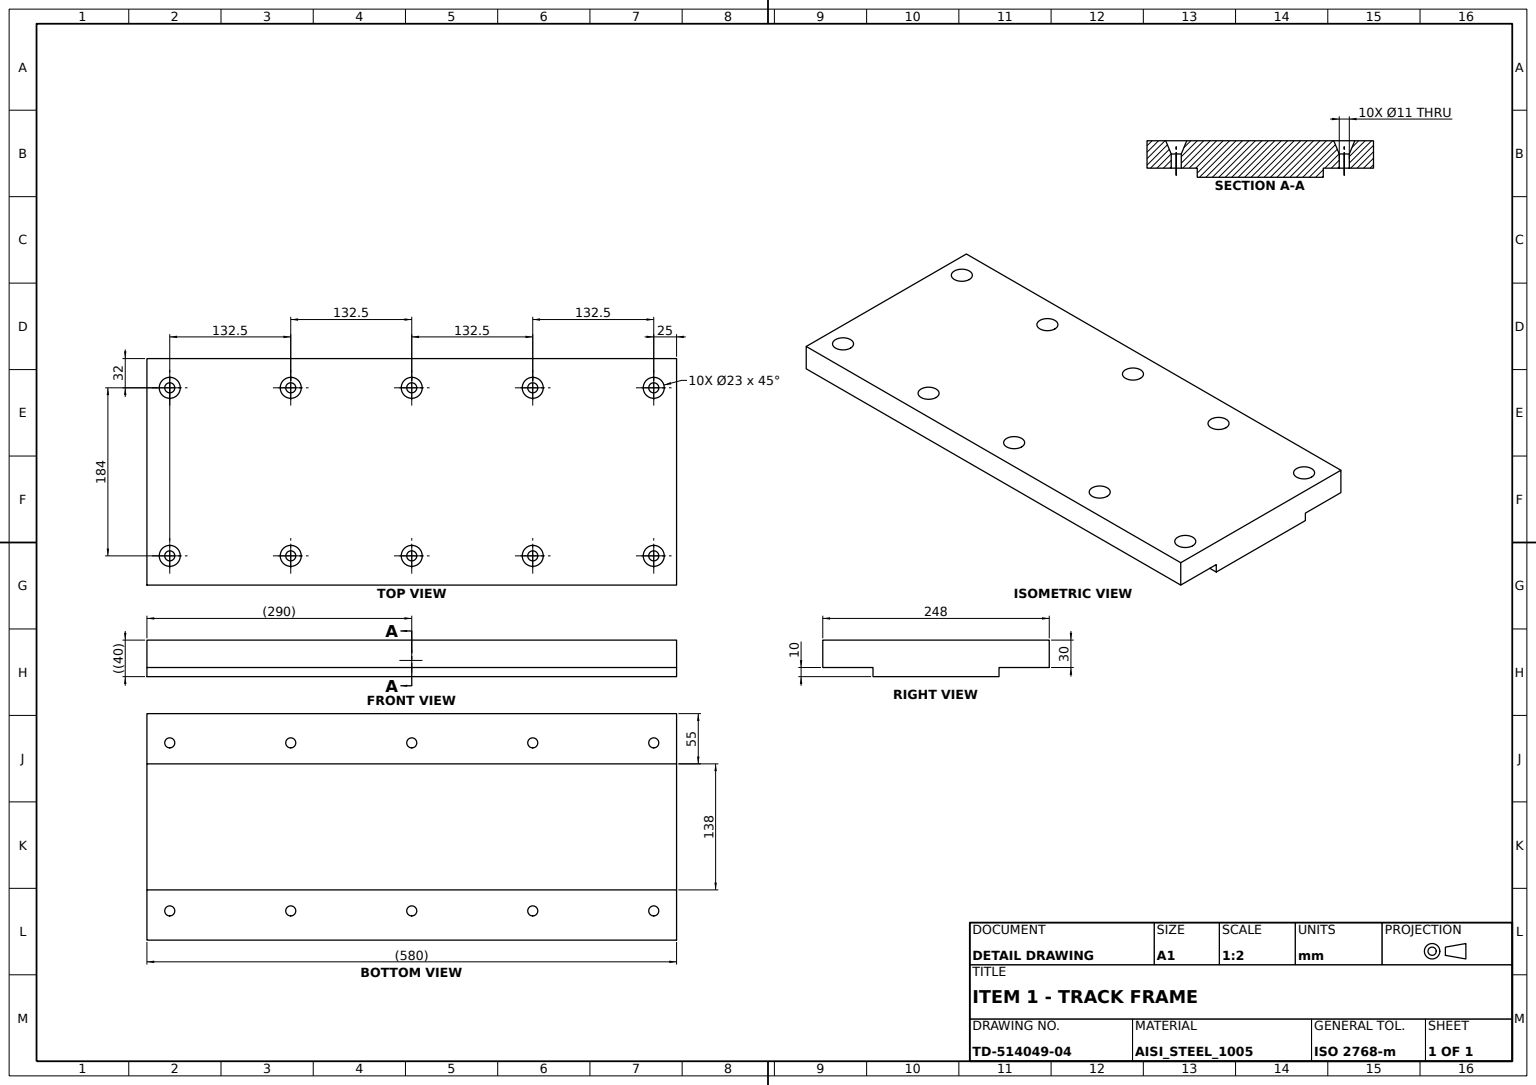
ISO-10303-21;
HEADER;
FILE_DESCRIPTION((''),'2;1');
FILE_NAME('','',(''),(''),'','','');
FILE_SCHEMA(('AUTOMOTIVE_DESIGN'));
ENDSEC;
DATA;
#1=APPLICATION_CONTEXT('');
#2=PRODUCT_CONTEXT('',#1,'mechanical');
#3=PRODUCT('','','',(#2));
#4=PRODUCT_DEFINITION_FORMATION('','',#3);
#5=PRODUCT_DEFINITION_CONTEXT('',#1,'design');
#6=PRODUCT_DEFINITION('','',#4,#5);
#7=PRODUCT_DEFINITION_SHAPE('','',#6);
#8=(LENGTH_UNIT()NAMED_UNIT(*)SI_UNIT(.MILLI.,.METRE.));
#9=(NAMED_UNIT(*)PLANE_ANGLE_UNIT()SI_UNIT($,.RADIAN.));
#10=(NAMED_UNIT(*)SI_UNIT($,.STERADIAN.)SOLID_ANGLE_UNIT());
#11=UNCERTAINTY_MEASURE_WITH_UNIT(LENGTH_MEASURE(0.005),#8,'distance_accuracy_value','');
#12=(GEOMETRIC_REPRESENTATION_CONTEXT(3)GLOBAL_UNCERTAINTY_ASSIGNED_CONTEXT((#11))GLOBAL_UNIT_ASSIGNED_CONTEXT((#8,#9,#10))REPRESENTATION_CONTEXT('',''));
#13=CARTESIAN_POINT('',(-97.5,0.,-132.5));
#14=VERTEX_POINT('',#13);
#15=CARTESIAN_POINT('',(-92.,0.,-132.5));
#16=DIRECTION('',(0.,1.,0.));
#17=DIRECTION('',(-1.,0.,0.));
#18=AXIS2_PLACEMENT_3D('',#15,#16,#17);
#19=CIRCLE('',#18,5.5);
#20=EDGE_CURVE('',#14,#14,#19,.T.);
#21=ORIENTED_EDGE('',*,*,#20,.F.);
#22=EDGE_LOOP('',(#21));
#23=FACE_BOUND('',#22,.T.);
#24=CARTESIAN_POINT('',(-92.,15.514719,-138.));
#25=VERTEX_POINT('',#24);
#26=CARTESIAN_POINT('',(-92.,15.514719,-132.5));
#27=DIRECTION('',(0.,-1.,0.));
#28=DIRECTION('',(0.,0.,-1.));
#29=AXIS2_PLACEMENT_3D('',#26,#27,#28);
#30=CIRCLE('',#29,5.5);
#31=EDGE_CURVE('',#25,#25,#30,.F.);
#32=ORIENTED_EDGE('',*,*,#31,.T.);
#33=EDGE_LOOP('',(#32));
#34=FACE_BOUND('',#33,.T.);
#35=CARTESIAN_POINT('',(-92.,-494999.973717,-132.5));
#36=AXIS2_PLACEMENT_3D('',#35,#27,#28);
#37=CYLINDRICAL_SURFACE('',#36,5.5);
#38=ADVANCED_FACE('',(#23,#34),#37,.F.);
#39=CARTESIAN_POINT('',(92.,15.514719,259.5));
#40=VERTEX_POINT('',#39);
#41=CARTESIAN_POINT('',(92.,15.514719,265.));
#42=AXIS2_PLACEMENT_3D('',#41,#27,#28);
#43=CIRCLE('',#42,5.5);
#44=EDGE_CURVE('',#40,#40,#43,.F.);
#45=ORIENTED_EDGE('',*,*,#44,.F.);
#46=EDGE_LOOP('',(#45));
#47=FACE_BOUND('',#46,.T.);
#48=CARTESIAN_POINT('',(92.,30.,253.5));
#49=VERTEX_POINT('',#48);
#50=CARTESIAN_POINT('',(92.,30.,265.));
#51=AXIS2_PLACEMENT_3D('',#50,#27,#28);
#52=CIRCLE('',#51,11.5);
#53=EDGE_CURVE('',#49,#49,#52,.T.);
#54=ORIENTED_EDGE('',*,*,#53,.F.);
#55=EDGE_LOOP('',(#54));
#56=FACE_BOUND('',#55,.T.);
#57=DIRECTION('',(0.,0.,1.));
#58=AXIS2_PLACEMENT_3D('',#50,#16,#57);
#59=CONICAL_SURFACE('',#58,11.5,0.392699082);
#60=ADVANCED_FACE('',(#47,#56),#59,.F.);
#61=CARTESIAN_POINT('',(92.,15.514719,-138.));
#62=VERTEX_POINT('',#61);
#63=CARTESIAN_POINT('',(92.,15.514719,-132.5));
#64=AXIS2_PLACEMENT_3D('',#63,#27,#28);
#65=CIRCLE('',#64,5.5);
#66=EDGE_CURVE('',#62,#62,#65,.F.);
#67=ORIENTED_EDGE('',*,*,#66,.F.);
#68=EDGE_LOOP('',(#67));
#69=FACE_BOUND('',#68,.T.);
#70=CARTESIAN_POINT('',(92.,30.,-144.));
#71=VERTEX_POINT('',#70);
#72=CARTESIAN_POINT('',(92.,30.,-132.5));
#73=AXIS2_PLACEMENT_3D('',#72,#27,#28);
#74=CIRCLE('',#73,11.5);
#75=EDGE_CURVE('',#71,#71,#74,.T.);
#76=ORIENTED_EDGE('',*,*,#75,.F.);
#77=EDGE_LOOP('',(#76));
#78=FACE_BOUND('',#77,.T.);
#79=AXIS2_PLACEMENT_3D('',#72,#16,#57);
#80=CONICAL_SURFACE('',#79,11.5,0.392699082);
#81=ADVANCED_FACE('',(#69,#78),#80,.F.);
#82=CARTESIAN_POINT('',(86.5,0.,132.5));
#83=VERTEX_POINT('',#82);
#84=CARTESIAN_POINT('',(92.,0.,132.5));
#85=AXIS2_PLACEMENT_3D('',#84,#16,#17);
#86=CIRCLE('',#85,5.5);
#87=EDGE_CURVE('',#83,#83,#86,.T.);
#88=ORIENTED_EDGE('',*,*,#87,.F.);
#89=EDGE_LOOP('',(#88));
#90=FACE_BOUND('',#89,.T.);
#91=CARTESIAN_POINT('',(92.,15.514719,127.));
#92=VERTEX_POINT('',#91);
#93=CARTESIAN_POINT('',(92.,15.514719,132.5));
#94=AXIS2_PLACEMENT_3D('',#93,#27,#28);
#95=CIRCLE('',#94,5.5);
#96=EDGE_CURVE('',#92,#92,#95,.F.);
#97=ORIENTED_EDGE('',*,*,#96,.T.);
#98=EDGE_LOOP('',(#97));
#99=FACE_BOUND('',#98,.T.);
#100=CARTESIAN_POINT('',(92.,-494999.973717,132.5));
#101=AXIS2_PLACEMENT_3D('',#100,#27,#28);
#102=CYLINDRICAL_SURFACE('',#101,5.5);
#103=ADVANCED_FACE('',(#90,#99),#102,.F.);
#104=CARTESIAN_POINT('',(124.,0.,290.));
#105=VERTEX_POINT('',#104);
#106=CARTESIAN_POINT('',(124.,30.,290.));
#107=VERTEX_POINT('',#106);
#108=VECTOR('',#16,1000.);
#109=LINE('',#104,#108);
#110=EDGE_CURVE('',#105,#107,#109,.T.);
#111=ORIENTED_EDGE('',*,*,#110,.F.);
#112=CARTESIAN_POINT('',(124.,0.,-290.));
#113=VERTEX_POINT('',#112);
#114=VECTOR('',#28,1000.);
#115=LINE('',#104,#114);
#116=EDGE_CURVE('',#105,#113,#115,.T.);
#117=ORIENTED_EDGE('',*,*,#116,.T.);
#118=CARTESIAN_POINT('',(124.,30.,-290.));
#119=VERTEX_POINT('',#118);
#120=LINE('',#112,#108);
#121=EDGE_CURVE('',#113,#119,#120,.T.);
#122=ORIENTED_EDGE('',*,*,#121,.T.);
#123=LINE('',#106,#114);
#124=EDGE_CURVE('',#107,#119,#123,.T.);
#125=ORIENTED_EDGE('',*,*,#124,.F.);
#126=EDGE_LOOP('',(#111,#117,#122,#125));
#127=FACE_BOUND('',#126,.T.);
#128=AXIS2_PLACEMENT_3D('',#104,#17,#57);
#129=PLANE('',#128);
#130=ADVANCED_FACE('',(#127),#129,.F.);
#131=CARTESIAN_POINT('',(-69.,0.,-290.));
#132=VERTEX_POINT('',#131);
#133=CARTESIAN_POINT('',(-69.,-10.,-290.));
#134=VERTEX_POINT('',#133);
#135=VECTOR('',#27,1000.);
#136=LINE('',#131,#135);
#137=EDGE_CURVE('',#132,#134,#136,.T.);
#138=ORIENTED_EDGE('',*,*,#137,.T.);
#139=CARTESIAN_POINT('',(-69.,-10.,290.));
#140=VERTEX_POINT('',#139);
#141=LINE('',#139,#114);
#142=EDGE_CURVE('',#140,#134,#141,.T.);
#143=ORIENTED_EDGE('',*,*,#142,.F.);
#144=CARTESIAN_POINT('',(-69.,0.,290.));
#145=VERTEX_POINT('',#144);
#146=LINE('',#144,#135);
#147=EDGE_CURVE('',#145,#140,#146,.T.);
#148=ORIENTED_EDGE('',*,*,#147,.F.);
#149=LINE('',#144,#114);
#150=EDGE_CURVE('',#145,#132,#149,.T.);
#151=ORIENTED_EDGE('',*,*,#150,.T.);
#152=EDGE_LOOP('',(#138,#143,#148,#151));
#153=FACE_BOUND('',#152,.T.);
#154=DIRECTION('',(1.,0.,0.));
#155=AXIS2_PLACEMENT_3D('',#144,#154,#28);
#156=PLANE('',#155);
#157=ADVANCED_FACE('',(#153),#156,.F.);
#158=CARTESIAN_POINT('',(-92.,30.,-144.));
#159=VERTEX_POINT('',#158);
#160=CARTESIAN_POINT('',(-92.,30.,-132.5));
#161=AXIS2_PLACEMENT_3D('',#160,#27,#28);
#162=CIRCLE('',#161,11.5);
#163=EDGE_CURVE('',#159,#159,#162,.T.);
#164=ORIENTED_EDGE('',*,*,#163,.F.);
#165=EDGE_LOOP('',(#164));
#166=FACE_BOUND('',#165,.T.);
#167=ORIENTED_EDGE('',*,*,#31,.F.);
#168=EDGE_LOOP('',(#167));
#169=FACE_BOUND('',#168,.T.);
#170=AXIS2_PLACEMENT_3D('',#160,#16,#57);
#171=CONICAL_SURFACE('',#170,11.5,0.392699082);
#172=ADVANCED_FACE('',(#166,#169),#171,.F.);
#173=CARTESIAN_POINT('',(-124.,30.,-290.));
#174=VERTEX_POINT('',#173);
#175=CARTESIAN_POINT('',(-124.,0.,-290.));
#176=VERTEX_POINT('',#175);
#177=LINE('',#173,#135);
#178=EDGE_CURVE('',#174,#176,#177,.T.);
#179=ORIENTED_EDGE('',*,*,#178,.F.);
#180=VECTOR('',#17,1000.);
#181=LINE('',#118,#180);
#182=EDGE_CURVE('',#119,#174,#181,.T.);
#183=ORIENTED_EDGE('',*,*,#182,.F.);
#184=ORIENTED_EDGE('',*,*,#121,.F.);
#185=CARTESIAN_POINT('',(69.,0.,-290.));
#186=VERTEX_POINT('',#185);
#187=VECTOR('',#154,1000.);
#188=LINE('',#185,#187);
#189=EDGE_CURVE('',#186,#113,#188,.T.);
#190=ORIENTED_EDGE('',*,*,#189,.F.);
#191=CARTESIAN_POINT('',(69.,-10.,-290.));
#192=VERTEX_POINT('',#191);
#193=LINE('',#191,#108);
#194=EDGE_CURVE('',#192,#186,#193,.T.);
#195=ORIENTED_EDGE('',*,*,#194,.F.);
#196=LINE('',#133,#187);
#197=EDGE_CURVE('',#134,#192,#196,.T.);
#198=ORIENTED_EDGE('',*,*,#197,.F.);
#199=ORIENTED_EDGE('',*,*,#137,.F.);
#200=LINE('',#175,#187);
#201=EDGE_CURVE('',#176,#132,#200,.T.);
#202=ORIENTED_EDGE('',*,*,#201,.F.);
#203=EDGE_LOOP('',(#179,#183,#184,#190,#195,#198,#199,#202));
#204=FACE_BOUND('',#203,.T.);
#205=CARTESIAN_POINT('',(0.,0.,-290.));
#206=AXIS2_PLACEMENT_3D('',#205,#28,#17);
#207=PLANE('',#206);
#208=ADVANCED_FACE('',(#204),#207,.T.);
#209=CARTESIAN_POINT('',(86.5,0.,265.));
#210=VERTEX_POINT('',#209);
#211=CARTESIAN_POINT('',(92.,0.,265.));
#212=AXIS2_PLACEMENT_3D('',#211,#16,#17);
#213=CIRCLE('',#212,5.5);
#214=EDGE_CURVE('',#210,#210,#213,.T.);
#215=ORIENTED_EDGE('',*,*,#214,.F.);
#216=EDGE_LOOP('',(#215));
#217=FACE_BOUND('',#216,.T.);
#218=ORIENTED_EDGE('',*,*,#44,.T.);
#219=EDGE_LOOP('',(#218));
#220=FACE_BOUND('',#219,.T.);
#221=CARTESIAN_POINT('',(92.,-494999.920516,265.));
#222=AXIS2_PLACEMENT_3D('',#221,#27,#28);
#223=CYLINDRICAL_SURFACE('',#222,5.5);
#224=ADVANCED_FACE('',(#217,#220),#223,.F.);
#225=CARTESIAN_POINT('',(-92.,15.514719,-270.5));
#226=VERTEX_POINT('',#225);
#227=CARTESIAN_POINT('',(-92.,15.514719,-265.));
#228=AXIS2_PLACEMENT_3D('',#227,#27,#28);
#229=CIRCLE('',#228,5.5);
#230=EDGE_CURVE('',#226,#226,#229,.F.);
#231=ORIENTED_EDGE('',*,*,#230,.T.);
#232=EDGE_LOOP('',(#231));
#233=FACE_BOUND('',#232,.T.);
#234=CARTESIAN_POINT('',(-97.5,0.,-265.));
#235=VERTEX_POINT('',#234);
#236=CARTESIAN_POINT('',(-92.,0.,-265.));
#237=AXIS2_PLACEMENT_3D('',#236,#16,#17);
#238=CIRCLE('',#237,5.5);
#239=EDGE_CURVE('',#235,#235,#238,.T.);
#240=ORIENTED_EDGE('',*,*,#239,.F.);
#241=EDGE_LOOP('',(#240));
#242=FACE_BOUND('',#241,.T.);
#243=CARTESIAN_POINT('',(-92.,-494999.920516,-265.));
#244=AXIS2_PLACEMENT_3D('',#243,#27,#28);
#245=CYLINDRICAL_SURFACE('',#244,5.5);
#246=ADVANCED_FACE('',(#233,#242),#245,.F.);
#247=CARTESIAN_POINT('',(92.,15.514719,-5.5));
#248=VERTEX_POINT('',#247);
#249=CARTESIAN_POINT('',(92.,15.514719,0.));
#250=AXIS2_PLACEMENT_3D('',#249,#27,#28);
#251=CIRCLE('',#250,5.5);
#252=EDGE_CURVE('',#248,#248,#251,.F.);
#253=ORIENTED_EDGE('',*,*,#252,.T.);
#254=EDGE_LOOP('',(#253));
#255=FACE_BOUND('',#254,.T.);
#256=CARTESIAN_POINT('',(86.5,0.,0.));
#257=VERTEX_POINT('',#256);
#258=CARTESIAN_POINT('',(92.,0.,0.));
#259=AXIS2_PLACEMENT_3D('',#258,#16,#17);
#260=CIRCLE('',#259,5.5);
#261=EDGE_CURVE('',#257,#257,#260,.T.);
#262=ORIENTED_EDGE('',*,*,#261,.F.);
#263=EDGE_LOOP('',(#262));
#264=FACE_BOUND('',#263,.T.);
#265=CARTESIAN_POINT('',(92.,-494999.991451,0.));
#266=AXIS2_PLACEMENT_3D('',#265,#27,#28);
#267=CYLINDRICAL_SURFACE('',#266,5.5);
#268=ADVANCED_FACE('',(#255,#264),#267,.F.);
#269=ORIENTED_EDGE('',*,*,#96,.F.);
#270=EDGE_LOOP('',(#269));
#271=FACE_BOUND('',#270,.T.);
#272=CARTESIAN_POINT('',(92.,30.,121.));
#273=VERTEX_POINT('',#272);
#274=CARTESIAN_POINT('',(92.,30.,132.5));
#275=AXIS2_PLACEMENT_3D('',#274,#27,#28);
#276=CIRCLE('',#275,11.5);
#277=EDGE_CURVE('',#273,#273,#276,.T.);
#278=ORIENTED_EDGE('',*,*,#277,.F.);
#279=EDGE_LOOP('',(#278));
#280=FACE_BOUND('',#279,.T.);
#281=AXIS2_PLACEMENT_3D('',#274,#16,#57);
#282=CONICAL_SURFACE('',#281,11.5,0.392699082);
#283=ADVANCED_FACE('',(#271,#280),#282,.F.);
#284=CARTESIAN_POINT('',(-92.,30.,-276.5));
#285=VERTEX_POINT('',#284);
#286=CARTESIAN_POINT('',(-92.,30.,-265.));
#287=AXIS2_PLACEMENT_3D('',#286,#27,#28);
#288=CIRCLE('',#287,11.5);
#289=EDGE_CURVE('',#285,#285,#288,.T.);
#290=ORIENTED_EDGE('',*,*,#289,.F.);
#291=EDGE_LOOP('',(#290));
#292=FACE_BOUND('',#291,.T.);
#293=ORIENTED_EDGE('',*,*,#230,.F.);
#294=EDGE_LOOP('',(#293));
#295=FACE_BOUND('',#294,.T.);
#296=AXIS2_PLACEMENT_3D('',#286,#16,#57);
#297=CONICAL_SURFACE('',#296,11.5,0.392699082);
#298=ADVANCED_FACE('',(#292,#295),#297,.F.);
#299=CARTESIAN_POINT('',(-92.,30.,-11.5));
#300=VERTEX_POINT('',#299);
#301=CARTESIAN_POINT('',(-92.,30.,0.));
#302=AXIS2_PLACEMENT_3D('',#301,#27,#28);
#303=CIRCLE('',#302,11.5);
#304=EDGE_CURVE('',#300,#300,#303,.T.);
#305=ORIENTED_EDGE('',*,*,#304,.T.);
#306=EDGE_LOOP('',(#305));
#307=FACE_BOUND('',#306,.T.);
#308=ORIENTED_EDGE('',*,*,#289,.T.);
#309=EDGE_LOOP('',(#308));
#310=FACE_BOUND('',#309,.T.);
#311=CARTESIAN_POINT('',(-124.,30.,290.));
#312=VERTEX_POINT('',#311);
#313=LINE('',#106,#180);
#314=EDGE_CURVE('',#107,#312,#313,.T.);
#315=ORIENTED_EDGE('',*,*,#314,.F.);
#316=ORIENTED_EDGE('',*,*,#124,.T.);
#317=ORIENTED_EDGE('',*,*,#182,.T.);
#318=LINE('',#311,#114);
#319=EDGE_CURVE('',#312,#174,#318,.T.);
#320=ORIENTED_EDGE('',*,*,#319,.F.);
#321=EDGE_LOOP('',(#315,#316,#317,#320));
#322=FACE_BOUND('',#321,.T.);
#323=ORIENTED_EDGE('',*,*,#53,.T.);
#324=EDGE_LOOP('',(#323));
#325=FACE_BOUND('',#324,.T.);
#326=ORIENTED_EDGE('',*,*,#163,.T.);
#327=EDGE_LOOP('',(#326));
#328=FACE_BOUND('',#327,.T.);
#329=CARTESIAN_POINT('',(92.,30.,-276.5));
#330=VERTEX_POINT('',#329);
#331=CARTESIAN_POINT('',(92.,30.,-265.));
#332=AXIS2_PLACEMENT_3D('',#331,#27,#28);
#333=CIRCLE('',#332,11.5);
#334=EDGE_CURVE('',#330,#330,#333,.T.);
#335=ORIENTED_EDGE('',*,*,#334,.T.);
#336=EDGE_LOOP('',(#335));
#337=FACE_BOUND('',#336,.T.);
#338=CARTESIAN_POINT('',(92.,30.,-11.5));
#339=VERTEX_POINT('',#338);
#340=CARTESIAN_POINT('',(92.,30.,0.));
#341=AXIS2_PLACEMENT_3D('',#340,#27,#28);
#342=CIRCLE('',#341,11.5);
#343=EDGE_CURVE('',#339,#339,#342,.T.);
#344=ORIENTED_EDGE('',*,*,#343,.T.);
#345=EDGE_LOOP('',(#344));
#346=FACE_BOUND('',#345,.T.);
#347=CARTESIAN_POINT('',(-92.,30.,121.));
#348=VERTEX_POINT('',#347);
#349=CARTESIAN_POINT('',(-92.,30.,132.5));
#350=AXIS2_PLACEMENT_3D('',#349,#27,#28);
#351=CIRCLE('',#350,11.5);
#352=EDGE_CURVE('',#348,#348,#351,.T.);
#353=ORIENTED_EDGE('',*,*,#352,.T.);
#354=EDGE_LOOP('',(#353));
#355=FACE_BOUND('',#354,.T.);
#356=ORIENTED_EDGE('',*,*,#277,.T.);
#357=EDGE_LOOP('',(#356));
#358=FACE_BOUND('',#357,.T.);
#359=CARTESIAN_POINT('',(-92.,30.,253.5));
#360=VERTEX_POINT('',#359);
#361=CARTESIAN_POINT('',(-92.,30.,265.));
#362=AXIS2_PLACEMENT_3D('',#361,#27,#28);
#363=CIRCLE('',#362,11.5);
#364=EDGE_CURVE('',#360,#360,#363,.T.);
#365=ORIENTED_EDGE('',*,*,#364,.T.);
#366=EDGE_LOOP('',(#365));
#367=FACE_BOUND('',#366,.T.);
#368=ORIENTED_EDGE('',*,*,#75,.T.);
#369=EDGE_LOOP('',(#368));
#370=FACE_BOUND('',#369,.T.);
#371=AXIS2_PLACEMENT_3D('',#106,#27,#28);
#372=PLANE('',#371);
#373=ADVANCED_FACE('',(#307,#310,#322,#325,#328,#337,#346,#355,#358,#367,#370),#372,.F.);
#374=ORIENTED_EDGE('',*,*,#319,.T.);
#375=ORIENTED_EDGE('',*,*,#178,.T.);
#376=CARTESIAN_POINT('',(-124.,0.,290.));
#377=VERTEX_POINT('',#376);
#378=LINE('',#376,#114);
#379=EDGE_CURVE('',#377,#176,#378,.T.);
#380=ORIENTED_EDGE('',*,*,#379,.F.);
#381=LINE('',#311,#135);
#382=EDGE_CURVE('',#312,#377,#381,.T.);
#383=ORIENTED_EDGE('',*,*,#382,.F.);
#384=EDGE_LOOP('',(#374,#375,#380,#383));
#385=FACE_BOUND('',#384,.T.);
#386=AXIS2_PLACEMENT_3D('',#311,#154,#28);
#387=PLANE('',#386);
#388=ADVANCED_FACE('',(#385),#387,.F.);
#389=CARTESIAN_POINT('',(-97.5,0.,0.));
#390=VERTEX_POINT('',#389);
#391=CARTESIAN_POINT('',(-92.,0.,0.));
#392=AXIS2_PLACEMENT_3D('',#391,#16,#17);
#393=CIRCLE('',#392,5.5);
#394=EDGE_CURVE('',#390,#390,#393,.T.);
#395=ORIENTED_EDGE('',*,*,#394,.F.);
#396=EDGE_LOOP('',(#395));
#397=FACE_BOUND('',#396,.T.);
#398=CARTESIAN_POINT('',(-92.,15.514719,-5.5));
#399=VERTEX_POINT('',#398);
#400=CARTESIAN_POINT('',(-92.,15.514719,0.));
#401=AXIS2_PLACEMENT_3D('',#400,#27,#28);
#402=CIRCLE('',#401,5.5);
#403=EDGE_CURVE('',#399,#399,#402,.F.);
#404=ORIENTED_EDGE('',*,*,#403,.T.);
#405=EDGE_LOOP('',(#404));
#406=FACE_BOUND('',#405,.T.);
#407=CARTESIAN_POINT('',(-92.,-494999.991451,0.));
#408=AXIS2_PLACEMENT_3D('',#407,#27,#28);
#409=CYLINDRICAL_SURFACE('',#408,5.5);
#410=ADVANCED_FACE('',(#397,#406),#409,.F.);
#411=CARTESIAN_POINT('',(-97.5,0.,132.5));
#412=VERTEX_POINT('',#411);
#413=CARTESIAN_POINT('',(-92.,0.,132.5));
#414=AXIS2_PLACEMENT_3D('',#413,#16,#17);
#415=CIRCLE('',#414,5.5);
#416=EDGE_CURVE('',#412,#412,#415,.T.);
#417=ORIENTED_EDGE('',*,*,#416,.F.);
#418=EDGE_LOOP('',(#417));
#419=FACE_BOUND('',#418,.T.);
#420=CARTESIAN_POINT('',(-92.,15.514719,127.));
#421=VERTEX_POINT('',#420);
#422=CARTESIAN_POINT('',(-92.,15.514719,132.5));
#423=AXIS2_PLACEMENT_3D('',#422,#27,#28);
#424=CIRCLE('',#423,5.5);
#425=EDGE_CURVE('',#421,#421,#424,.F.);
#426=ORIENTED_EDGE('',*,*,#425,.T.);
#427=EDGE_LOOP('',(#426));
#428=FACE_BOUND('',#427,.T.);
#429=CARTESIAN_POINT('',(-92.,-494999.973717,132.5));
#430=AXIS2_PLACEMENT_3D('',#429,#27,#28);
#431=CYLINDRICAL_SURFACE('',#430,5.5);
#432=ADVANCED_FACE('',(#419,#428),#431,.F.);
#433=ORIENTED_EDGE('',*,*,#194,.T.);
#434=CARTESIAN_POINT('',(69.,0.,290.));
#435=VERTEX_POINT('',#434);
#436=LINE('',#434,#114);
#437=EDGE_CURVE('',#435,#186,#436,.T.);
#438=ORIENTED_EDGE('',*,*,#437,.F.);
#439=CARTESIAN_POINT('',(69.,-10.,290.));
#440=VERTEX_POINT('',#439);
#441=LINE('',#439,#108);
#442=EDGE_CURVE('',#440,#435,#441,.T.);
#443=ORIENTED_EDGE('',*,*,#442,.F.);
#444=LINE('',#439,#114);
#445=EDGE_CURVE('',#440,#192,#444,.T.);
#446=ORIENTED_EDGE('',*,*,#445,.T.);
#447=EDGE_LOOP('',(#433,#438,#443,#446));
#448=FACE_BOUND('',#447,.T.);
#449=AXIS2_PLACEMENT_3D('',#439,#17,#57);
#450=PLANE('',#449);
#451=ADVANCED_FACE('',(#448),#450,.F.);
#452=ORIENTED_EDGE('',*,*,#252,.F.);
#453=EDGE_LOOP('',(#452));
#454=FACE_BOUND('',#453,.T.);
#455=ORIENTED_EDGE('',*,*,#343,.F.);
#456=EDGE_LOOP('',(#455));
#457=FACE_BOUND('',#456,.T.);
#458=AXIS2_PLACEMENT_3D('',#340,#16,#57);
#459=CONICAL_SURFACE('',#458,11.5,0.392699082);
#460=ADVANCED_FACE('',(#454,#457),#459,.F.);
#461=ORIENTED_EDGE('',*,*,#403,.F.);
#462=EDGE_LOOP('',(#461));
#463=FACE_BOUND('',#462,.T.);
#464=ORIENTED_EDGE('',*,*,#304,.F.);
#465=EDGE_LOOP('',(#464));
#466=FACE_BOUND('',#465,.T.);
#467=AXIS2_PLACEMENT_3D('',#301,#16,#57);
#468=CONICAL_SURFACE('',#467,11.5,0.392699082);
#469=ADVANCED_FACE('',(#463,#466),#468,.F.);
#470=CARTESIAN_POINT('',(86.5,0.,-132.5));
#471=VERTEX_POINT('',#470);
#472=CARTESIAN_POINT('',(92.,0.,-132.5));
#473=AXIS2_PLACEMENT_3D('',#472,#16,#17);
#474=CIRCLE('',#473,5.5);
#475=EDGE_CURVE('',#471,#471,#474,.T.);
#476=ORIENTED_EDGE('',*,*,#475,.T.);
#477=EDGE_LOOP('',(#476));
#478=FACE_BOUND('',#477,.T.);
#479=ORIENTED_EDGE('',*,*,#87,.T.);
#480=EDGE_LOOP('',(#479));
#481=FACE_BOUND('',#480,.T.);
#482=ORIENTED_EDGE('',*,*,#261,.T.);
#483=EDGE_LOOP('',(#482));
#484=FACE_BOUND('',#483,.T.);
#485=LINE('',#434,#187);
#486=EDGE_CURVE('',#435,#105,#485,.T.);
#487=ORIENTED_EDGE('',*,*,#486,.F.);
#488=ORIENTED_EDGE('',*,*,#437,.T.);
#489=ORIENTED_EDGE('',*,*,#189,.T.);
#490=ORIENTED_EDGE('',*,*,#116,.F.);
#491=EDGE_LOOP('',(#487,#488,#489,#490));
#492=FACE_BOUND('',#491,.T.);
#493=ORIENTED_EDGE('',*,*,#214,.T.);
#494=EDGE_LOOP('',(#493));
#495=FACE_BOUND('',#494,.T.);
#496=CARTESIAN_POINT('',(86.5,0.,-265.));
#497=VERTEX_POINT('',#496);
#498=CARTESIAN_POINT('',(92.,0.,-265.));
#499=AXIS2_PLACEMENT_3D('',#498,#16,#17);
#500=CIRCLE('',#499,5.5);
#501=EDGE_CURVE('',#497,#497,#500,.T.);
#502=ORIENTED_EDGE('',*,*,#501,.T.);
#503=EDGE_LOOP('',(#502));
#504=FACE_BOUND('',#503,.T.);
#505=AXIS2_PLACEMENT_3D('',#434,#16,#17);
#506=PLANE('',#505);
#507=ADVANCED_FACE('',(#478,#481,#484,#492,#495,#504),#506,.F.);
#508=LINE('',#139,#187);
#509=EDGE_CURVE('',#140,#440,#508,.T.);
#510=ORIENTED_EDGE('',*,*,#509,.F.);
#511=ORIENTED_EDGE('',*,*,#142,.T.);
#512=ORIENTED_EDGE('',*,*,#197,.T.);
#513=ORIENTED_EDGE('',*,*,#445,.F.);
#514=EDGE_LOOP('',(#510,#511,#512,#513));
#515=FACE_BOUND('',#514,.T.);
#516=AXIS2_PLACEMENT_3D('',#139,#16,#17);
#517=PLANE('',#516);
#518=ADVANCED_FACE('',(#515),#517,.F.);
#519=ORIENTED_EDGE('',*,*,#425,.F.);
#520=EDGE_LOOP('',(#519));
#521=FACE_BOUND('',#520,.T.);
#522=ORIENTED_EDGE('',*,*,#352,.F.);
#523=EDGE_LOOP('',(#522));
#524=FACE_BOUND('',#523,.T.);
#525=AXIS2_PLACEMENT_3D('',#349,#16,#57);
#526=CONICAL_SURFACE('',#525,11.5,0.392699082);
#527=ADVANCED_FACE('',(#521,#524),#526,.F.);
#528=ORIENTED_EDGE('',*,*,#364,.F.);
#529=EDGE_LOOP('',(#528));
#530=FACE_BOUND('',#529,.T.);
#531=CARTESIAN_POINT('',(-92.,15.514719,259.5));
#532=VERTEX_POINT('',#531);
#533=CARTESIAN_POINT('',(-92.,15.514719,265.));
#534=AXIS2_PLACEMENT_3D('',#533,#27,#28);
#535=CIRCLE('',#534,5.5);
#536=EDGE_CURVE('',#532,#532,#535,.F.);
#537=ORIENTED_EDGE('',*,*,#536,.F.);
#538=EDGE_LOOP('',(#537));
#539=FACE_BOUND('',#538,.T.);
#540=AXIS2_PLACEMENT_3D('',#361,#16,#57);
#541=CONICAL_SURFACE('',#540,11.5,0.392699082);
#542=ADVANCED_FACE('',(#530,#539),#541,.F.);
#543=ORIENTED_EDGE('',*,*,#475,.F.);
#544=EDGE_LOOP('',(#543));
#545=FACE_BOUND('',#544,.T.);
#546=ORIENTED_EDGE('',*,*,#66,.T.);
#547=EDGE_LOOP('',(#546));
#548=FACE_BOUND('',#547,.T.);
#549=CARTESIAN_POINT('',(92.,-494999.973717,-132.5));
#550=AXIS2_PLACEMENT_3D('',#549,#27,#28);
#551=CYLINDRICAL_SURFACE('',#550,5.5);
#552=ADVANCED_FACE('',(#545,#548),#551,.F.);
#553=ORIENTED_EDGE('',*,*,#334,.F.);
#554=EDGE_LOOP('',(#553));
#555=FACE_BOUND('',#554,.T.);
#556=CARTESIAN_POINT('',(92.,15.514719,-270.5));
#557=VERTEX_POINT('',#556);
#558=CARTESIAN_POINT('',(92.,15.514719,-265.));
#559=AXIS2_PLACEMENT_3D('',#558,#27,#28);
#560=CIRCLE('',#559,5.5);
#561=EDGE_CURVE('',#557,#557,#560,.F.);
#562=ORIENTED_EDGE('',*,*,#561,.F.);
#563=EDGE_LOOP('',(#562));
#564=FACE_BOUND('',#563,.T.);
#565=AXIS2_PLACEMENT_3D('',#331,#16,#57);
#566=CONICAL_SURFACE('',#565,11.5,0.392699082);
#567=ADVANCED_FACE('',(#555,#564),#566,.F.);
#568=ORIENTED_EDGE('',*,*,#20,.T.);
#569=EDGE_LOOP('',(#568));
#570=FACE_BOUND('',#569,.T.);
#571=CARTESIAN_POINT('',(-97.5,0.,265.));
#572=VERTEX_POINT('',#571);
#573=CARTESIAN_POINT('',(-92.,0.,265.));
#574=AXIS2_PLACEMENT_3D('',#573,#16,#17);
#575=CIRCLE('',#574,5.5);
#576=EDGE_CURVE('',#572,#572,#575,.T.);
#577=ORIENTED_EDGE('',*,*,#576,.T.);
#578=EDGE_LOOP('',(#577));
#579=FACE_BOUND('',#578,.T.);
#580=ORIENTED_EDGE('',*,*,#394,.T.);
#581=EDGE_LOOP('',(#580));
#582=FACE_BOUND('',#581,.T.);
#583=LINE('',#376,#187);
#584=EDGE_CURVE('',#377,#145,#583,.T.);
#585=ORIENTED_EDGE('',*,*,#584,.F.);
#586=ORIENTED_EDGE('',*,*,#379,.T.);
#587=ORIENTED_EDGE('',*,*,#201,.T.);
#588=ORIENTED_EDGE('',*,*,#150,.F.);
#589=EDGE_LOOP('',(#585,#586,#587,#588));
#590=FACE_BOUND('',#589,.T.);
#591=ORIENTED_EDGE('',*,*,#416,.T.);
#592=EDGE_LOOP('',(#591));
#593=FACE_BOUND('',#592,.T.);
#594=ORIENTED_EDGE('',*,*,#239,.T.);
#595=EDGE_LOOP('',(#594));
#596=FACE_BOUND('',#595,.T.);
#597=AXIS2_PLACEMENT_3D('',#376,#16,#17);
#598=PLANE('',#597);
#599=ADVANCED_FACE('',(#570,#579,#582,#590,#593,#596),#598,.F.);
#600=ORIENTED_EDGE('',*,*,#576,.F.);
#601=EDGE_LOOP('',(#600));
#602=FACE_BOUND('',#601,.T.);
#603=ORIENTED_EDGE('',*,*,#536,.T.);
#604=EDGE_LOOP('',(#603));
#605=FACE_BOUND('',#604,.T.);
#606=CARTESIAN_POINT('',(-92.,-494999.920516,265.));
#607=AXIS2_PLACEMENT_3D('',#606,#27,#28);
#608=CYLINDRICAL_SURFACE('',#607,5.5);
#609=ADVANCED_FACE('',(#602,#605),#608,.F.);
#610=ORIENTED_EDGE('',*,*,#486,.T.);
#611=ORIENTED_EDGE('',*,*,#110,.T.);
#612=ORIENTED_EDGE('',*,*,#314,.T.);
#613=ORIENTED_EDGE('',*,*,#382,.T.);
#614=ORIENTED_EDGE('',*,*,#584,.T.);
#615=ORIENTED_EDGE('',*,*,#147,.T.);
#616=ORIENTED_EDGE('',*,*,#509,.T.);
#617=ORIENTED_EDGE('',*,*,#442,.T.);
#618=EDGE_LOOP('',(#610,#611,#612,#613,#614,#615,#616,#617));
#619=FACE_BOUND('',#618,.T.);
#620=CARTESIAN_POINT('',(0.,0.,290.));
#621=AXIS2_PLACEMENT_3D('',#620,#28,#17);
#622=PLANE('',#621);
#623=ADVANCED_FACE('',(#619),#622,.F.);
#624=ORIENTED_EDGE('',*,*,#561,.T.);
#625=EDGE_LOOP('',(#624));
#626=FACE_BOUND('',#625,.T.);
#627=ORIENTED_EDGE('',*,*,#501,.F.);
#628=EDGE_LOOP('',(#627));
#629=FACE_BOUND('',#628,.T.);
#630=CARTESIAN_POINT('',(92.,-494999.920516,-265.));
#631=AXIS2_PLACEMENT_3D('',#630,#27,#28);
#632=CYLINDRICAL_SURFACE('',#631,5.5);
#633=ADVANCED_FACE('',(#626,#629),#632,.F.);
#634=CLOSED_SHELL('',(#38,#60,#81,#103,#130,#157,#172,#208,#224,#246,#268,#283,#298,#373,#388,#410,#432,#451,#460,#469,#507,#518,#527,#542,#552,#567,#599,#609,#623,#633));
#635=MANIFOLD_SOLID_BREP('',#634);
#636=ADVANCED_BREP_SHAPE_REPRESENTATION('',(#635),#12);
#637=SHAPE_DEFINITION_REPRESENTATION(#7,#636);
ENDSEC;
END-ISO-10303-21;
